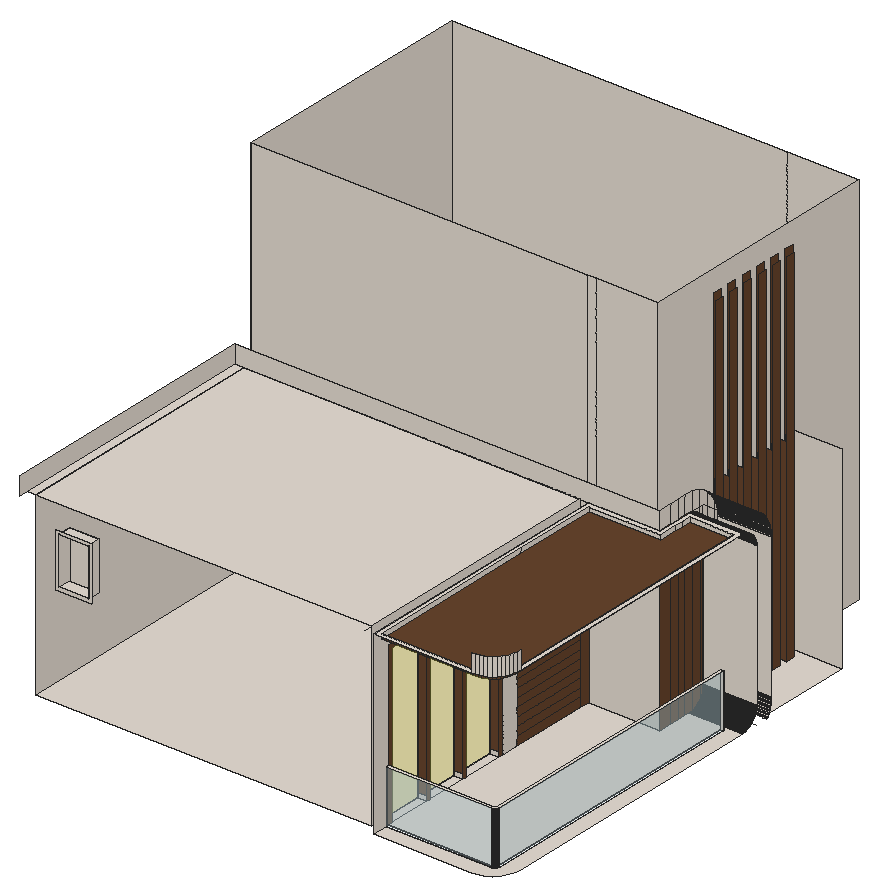
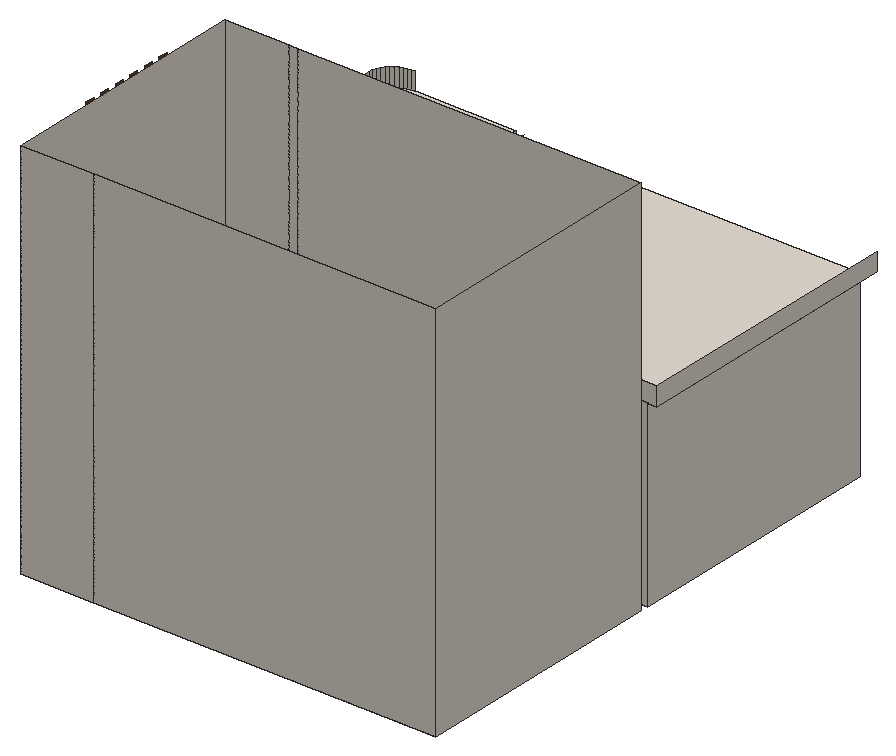
# SketchUp Ruby script. Lengths in inches.
U = 1.inch
M = Sketchup.active_model
def pt(a) = Geom::Point3d.new(a.map { |v| v * U })
def face(e, loops, mat)
  f = e.add_face(loops[0].map { |a| pt(a) })
  loops[1..].each { |l| e.add_face(l.map { |a| pt(a) }).erase! }
  f.material = f.back_material = mat if mat
  f
end
# faces: each face lists its corners as indices into pts; further lists are holes
def faces(e, pts, list, mat = nil) = list.each { |f| face(e, (f[0].is_a?(Array) ? f : [f]).map { |l| l.map { |i| pts[i] } }, mat) }
# xy, xz, yz: faces in a plane at the given z, y or x. An outline is a flat list of corners, or four numbers for a rectangle; further outlines are holes
def ring(l) = l.size == 4 ? [[l[0], l[1]], [l[2], l[1]], [l[2], l[3]], [l[0], l[3]]] : l.each_slice(2).to_a
def flat(e, list, mat, &to3) = list.each { |f| face(e, (f[0].is_a?(Array) ? f : [f]).map { |l| ring(l).map { |u, v| to3.(u, v) } }, mat) }
def xy(e, z, list, mat = nil) = flat(e, list, mat) { |x, y| [x, y, z] }
def xz(e, y, list, mat = nil) = flat(e, list, mat) { |x, z| [x, y, z] }
def yz(e, x, list, mat = nil) = flat(e, list, mat) { |y, z| [x, y, z] }
def lines(e, pts, list) = list.each { |a, b| e.add_line(pt(pts[a]), pt(pts[b])) }
# prism: a flat outline (further loops are holes) pulled along v
def prism(e, loops, v, mat = nil)
  f = face(e, loops, mat); d = Geom::Vector3d.new(v.map { |x| x * U })
  f.pushpull(f.normal.samedirection?(d) ? d.length : -d.length)
end
def box(e, o, s, mat = nil) = prism(e, [[o, [o[0] + s[0], o[1], o[2]], [o[0] + s[0], o[1] + s[1], o[2]], [o[0], o[1] + s[1], o[2]]]], [0, 0, s[2]], mat)
def at(x, y, z, deg = 0) = Geom::Transformation.translation(pt([x, y, z])) * Geom::Transformation.rotation(ORIGIN, Z_AXIS, deg.degrees)
def axes(o, x, y, z) = Geom::Transformation.new([*x, 0, *y, 0, *z, 0, *pt(o).to_a, 1])
def part(name) = M.definitions.add(name)
# library, detail: a bought-in or finely detailed component or shape, given as its bounding box
def library(name, o, s) = part(name).tap { |d| box(d.entities, o, s) }
def detail(e, o, s) = box(e.add_group.entities, o, s)
def put(e, d, t, mat = nil) = e.add_instance(d, t).tap { |i| i.material = mat if mat }
def group(e, t, mat = nil) = e.add_group.tap { |g| g.transformation = t; g.material = mat if mat }.entities
root = M.entities
M.materials.add("Glass_Basic_01").color = [255, 251, 32]
M.materials["Glass_Basic_01"].alpha = 0.25
M.materials.add("Glass_Safety_01").color = [204, 235, 244]
M.materials["Glass_Safety_01"].alpha = 0.25
M.materials.add("Marble_01_1K").color = [230, 221, 211]
M.materials.add("Wood_Veneer_15_1K").color = [103, 69, 45]
xy(root,132,[[273,36,339,36,341.36,36.13,343.68,36.57,345.92,37.3125,348.05,38.34,350.02,39.65,351.79,41.21,353.35,42.98,354.66,44.95,355.6875,47.08,356.43,49.32,356.87,51.64,357,54,357,240,321,240,321,216,273,216,273,48,344.08,48,344.21,48.02,344.33,48.0625,344.45,48.11,344.56,48.17,344.76,48.33,344.85,48.42,344.99,48.64,345.04,48.75,345.08,48.875,345.11,49,345.11,236.59,347.11,236.59,347.11,49,347.04,48.625,346.92,48.26,346.77,47.91,346.58,47.58,346.36,47.27,346.1,46.99,345.82,46.73,345.51,46.51,345.17,46.33,344.82,46.18,344.46,46.07,344.08,46,273,46],[42,42,267,216],[267,51,273,81],[267,83,273,111],[267,113,273,141],
  [42,222,315,390],[321,260.89,354,260.89,354,327,321,327,321,321,327,321,327,315,321,315,321,309,327,309,327,303,321,303,321,297,327,297,327,291,321,291,321,285,327,285,327,279,321,279,321,273,327,273,327,267,321,267],[321,267,327,273],[321,279,327,285],[321,291,327,297],
  [321,303,327,309],[321,315,327,321]],"Marble_01_1K")
xy(root,168,[[273,46,344.08,46,344.46,46.07,344.82,46.18,345.17,46.33,345.51,46.51,345.82,46.73,346.1,46.99,346.36,47.27,346.58,47.58,346.77,47.91,346.92,48.26,347.04,48.625,347.11,49,347.11,236.59,345.11,236.59,345.11,49,345.08,48.875,345.04,48.75,344.99,48.64,344.85,48.42,344.76,48.33,344.56,48.17,344.45,48.11,344.33,48.0625,344.21,48.02,344.08,48,273,48]],"Marble_01_1K")
xy(root,206,[[62,36,82,45]],"Marble_01_1K")
xy(root,237,[[267,51,273,81],[267,83,273,111],[267,113,273,141]],"Wood_Veneer_15_1K")
xy(root,238,[[62,36,82,45]],"Marble_01_1K")
xy(root,249,[[276,39,276,213,324,213,324,237,354,237,354,53.89,353.94,51.92,353.61,49.98,353.02,48.11,352.17,46.33,351.1,44.68,349.8,43.2,348.32,41.9,346.67,40.83,344.89,39.98,343.02,39.39,341.08,39.06,339.11,39]],"Wood_Veneer_15_1K")
xy(root,252,[[[273,36,273,216,321,216,321,240,357,240,357,54,356.92,51.62,356.53,49.28,355.81,47.01,354.79,44.86,353.49,42.87,351.92,41.08,350.13,39.51,348.14,38.21,345.99,37.19,343.72,36.47,341.38,36.08,339,36],[276,39,339.11,39,341.08,39.06,343.02,39.39,344.89,39.98,346.67,40.83,348.32,41.9,349.8,43.2,351.1,44.68,352.17,46.33,353.02,48.11,353.61,49.98,353.94,51.92,354,53.89,354,237,324,237,324,213,276,213]],[36,42,42,216],[42,42,267,216]],"Marble_01_1K")
xz(root,36,[[[60,204,84,240],[62,206,82,238]]],"Marble_01_1K")
xz(root,39,[[276,249,339.11,252]],"Wood_Veneer_15_1K")
xz(root,45,[[62,206,82,238]],"Marble_01_1K")
xz(root,46,[[273,132,344.08,168]],"Glass_Safety_01")
xz(root,48,[[273,132,344.08,168]],"Glass_Safety_01")
xz(root,51,[[267,132,273,135]],"Marble_01_1K")
xz(root,51,[[267,135,273,237]],"Wood_Veneer_15_1K")
xz(root,81,[[267,132,273,135]],"Marble_01_1K")
xz(root,81,[[267,135,273,237]],"Wood_Veneer_15_1K")
xz(root,83,[[267,132,273,135]],"Marble_01_1K")
xz(root,83,[[267,135,273,237]],"Wood_Veneer_15_1K")
xz(root,111,[[267,132,273,135]],"Marble_01_1K")
xz(root,111,[[267,135,273,237]],"Wood_Veneer_15_1K")
xz(root,113,[[267,132,273,135]],"Marble_01_1K")
xz(root,113,[[267,135,273,237]],"Wood_Veneer_15_1K")
xz(root,141,[[267,132,273,135]],"Marble_01_1K")
xz(root,141,[[267,135,273,237]],"Wood_Veneer_15_1K")
xz(root,213,[[276,249,324,252]],"Marble_01_1K")
xz(root,216,[[42,132,267,252],[273,132,321,252],[36,252,321,264]],"Marble_01_1K")
xz(root,222,[[42,132,267,384],[267,132,273,384],[273,132,315,384]],"Marble_01_1K")
xz(root,236.59,[[345.11,132,347.11,168]],"Marble_01_1K")
xz(root,237,[[324,249,354,252]],"Marble_01_1K")
xz(root,252,[[321,144,357,240]],"Marble_01_1K")
xz(root,261,[[321,251.14,327,264]],"Wood_Veneer_15_1K")
xz(root,264,[[321,143.24,357,144],[321,144,357,240]],"Marble_01_1K")
xz(root,267,[[321,132,327,264]],"Wood_Veneer_15_1K")
xz(root,273,[[321,132,327,264]],"Wood_Veneer_15_1K")
xz(root,279,[[321,132,327,264]],"Wood_Veneer_15_1K")
xz(root,285,[[321,132,327,264]],"Wood_Veneer_15_1K")
xz(root,291,[[321,132,327,264]],"Wood_Veneer_15_1K")
xz(root,297,[[321,132,327,264]],"Wood_Veneer_15_1K")
xz(root,303,[[321,132,327,264]],"Wood_Veneer_15_1K")
xz(root,309,[[321,132,327,264]],"Wood_Veneer_15_1K")
xz(root,315,[[321,132,327,264]],"Wood_Veneer_15_1K")
xz(root,321,[[321,132,327,264]],"Wood_Veneer_15_1K")
xz(root,327,[[321,132,354,264]],"Marble_01_1K")
xz(root,390,[[42,132,267,384],[267,132,315,384]],"Marble_01_1K")
yz(root,36,[[36,252,216,264]],"Marble_01_1K")
yz(root,42,[[42,132,216,252],[222,132,390,384]],"Marble_01_1K")
yz(root,62,[[36,206,45,238]],"Marble_01_1K")
yz(root,82,[[36,206,45,238]],"Marble_01_1K")
yz(root,267,[[51,132,81,237],[83,132,111,237],[113,132,141,237]],"Glass_Basic_01")
yz(root,267,[[42,132,42,252,216,252,216,132,141,132,141,237,113,237,113,132,111,132,111,237,83,237,83,132,81,132,81,237,51,237,51,132]],"Marble_01_1K")
yz(root,273,[[36,132,46,132,46,168,48,168,48,240,144,240,144,132,156,132,156,252,36,252]],"Marble_01_1K")
yz(root,273,[[48,132,51,132,51,237,141,237,141,132,144,132,144,240,48,240],[81,132,83,237],[111,132,113,237],[156,132,210,137.71],[210,132,216,132,216,252,156,252,156,246.26,210,246.26],
  [156,137.71,210,143.43],[156,143.43,210,149.14],[156,149.14,210,154.85],[156,154.85,210,160.56],[156,160.56,210,166.28],
  [156,166.28,210,171.99],[156,171.99,210,177.7],[156,177.7,210,183.42],[156,183.42,210,189.13],[156,189.13,210,194.84],
  [156,194.84,210,200.55],[156,200.55,210,206.27],[156,206.27,210,211.98],[156,211.98,210,217.69],[156,217.69,210,223.41],
  [156,223.41,210,229.12],[156,229.12,210,234.83],[156,234.83,210,240.55],[156,240.55,210,246.26]],"Wood_Veneer_15_1K")
yz(root,276,[[39,249,156,252],[156,249,213,252]],"Marble_01_1K")
yz(root,315,[[222,132,390,384]],"Marble_01_1K")
yz(root,321,[[252,132,255,132,255,258.4,254.54,258.77,253.95,259.22,253.34,259.65,252.71,260.07,252.08,260.46,251.43,260.84,250.77,261.2,250.11,261.54,249.43,261.85,249,262.04,249,252,252,252],[255,132,260.89,132,261,132.2,261,251.14,260.84,251.43,260.46,252.08,260.07,252.71,259.65,253.34,259.22,253.95,258.77,254.54,258.3,255.125,257.81,255.69,257.3,256.25,256.78,256.78,256.25,257.3,255.69,257.81,255.125,258.3,255,258.4],[260.89,132,261,132,261,132.2],[261,132.2,261.11,132.39,261.46,133.06,261.79,133.74,262.09,134.43,262.38,135.13,262.64,135.84,262.88,136.55,263.1,137.28,263.3,138.01,263.47,138.74,263.62,139.49,263.74,140.23,263.84,140.98,263.92,141.73,263.97,142.49,264,143.24,264,240,263.97,240.75,263.91,241.49,263.84,242.24,263.74,242.98,263.62,243.72,263.47,244.45,263.31,245.18,263.12,245.91,262.91,246.625,262.68,247.34,262.42,248.04,262.15,248.74,261.85,249.43,261.54,250.11,261.2,250.77,261,251.14],[216,252,225,264],
  [225,252,231,264],[231,252,237,264],[237,252,243,252,243,263.74,242.98,263.74,242.24,263.84,241.49,263.91,240.75,263.97,240,264,237,264],[243,252,249,252,249,262.04,248.74,262.15,248.04,262.42,247.34,262.68,246.625,262.91,245.91,263.12,245.18,263.31,244.45,263.47,243.72,263.62,243,263.74]],"Marble_01_1K")
yz(root,321,[[216,132,225,252],[225,132,231,252],[231,132,237,252],[237,132,240,132,240.37,132.02,241.11,132.1,241.48,132.16,241.85,132.23,242.21,132.3,242.57,132.39,242.93,132.49,243,132.51,243,251.26,242.83,251.32,242.49,251.4375,242.14,251.55,241.79,251.65,241.44,251.74,241.08,251.82,240.72,251.89,240.36,251.95,240,252,237,252],[261,132,267,132,267,375,261,375,261,251.14,261.2,250.77,261.54,250.11,261.85,249.43,262.15,248.74,262.42,248.04,262.68,247.34,262.91,246.625,263.12,245.91,263.31,245.18,263.47,244.45,263.62,243.72,263.74,242.98,263.84,242.24,263.91,241.49,263.97,240.75,264,240,264,143.24,263.97,142.49,263.92,141.73,263.84,140.98,263.74,140.23,263.62,139.49,263.47,138.74,263.3,138.01,263.1,137.28,262.88,136.55,262.64,135.84,262.38,135.13,262.09,134.43,261.79,133.74,261.46,133.06,261.11,132.39,261,132.2],
  [273,132,279,375],[285,132,291,375],[297,132,303,375],[309,132,315,375],[321,132,327,375],
  [243,132.51,243.29,132.6,243.64,132.72,243.99,132.85,244.33,132.99,244.67,133.14,245.01,133.3,245.34,133.47,245.66,133.65,245.98,133.84,246.3,134.04,246.61,134.25,246.91,134.47,247.2,134.69,247.78,135.17,248.05,135.42,248.32,135.68,248.58,135.95,248.83,136.22,249,136.42,249,246.97,248.78,247.24,248.54,247.51,248.29,247.78,248.04,248.04,247.78,248.29,247.51,248.54,247.24,248.78,246.95,249.02,246.67,249.24,246.375,249.46,246.08,249.67,245.77,249.875,245.47,250.07,244.83,250.43,244.51,250.6,243.85,250.92,243.52,251.06,243.18,251.2,243,251.26],[249,136.42,249.07,136.51,249.31,136.8,249.53,137.09,249.75,137.39,249.96,137.7,250.16,138.02,250.35,138.34,250.53,138.66,250.7,138.99,250.86,139.33,251.01,139.67,251.15,140.01,251.28,140.36,251.4,140.71,251.51,141.07,251.61,141.43,251.7,141.79,251.77,142.15,251.84,142.52,251.9,142.89,251.98,143.63,252,144,252,240,251.95,240.36,251.89,240.72,251.82,241.08,251.74,241.44,251.65,241.79,251.55,242.14,251.4375,242.49,251.32,242.83,251.2,243.18,251.06,243.52,250.92,243.85,250.6,244.51,250.43,244.83,250.07,245.47,249.875,245.77,249.67,246.08,249.46,246.375,249.24,246.67,249.02,246.95,249,246.97]],"Wood_Veneer_15_1K")
yz(root,324,[[213,249,225,252],[225,249,231,252],[231,249,237,252]],"Marble_01_1K")
yz(root,327,[[267,132,273,375],[279,132,285,375],[291,132,297,375],[303,132,309,375],[315,132,321,375],
  [261,251.14,261,375,255,375,255,258.4,255.125,258.3,255.69,257.81,256.25,257.3,256.78,256.78,257.3,256.25,257.81,255.69,258.3,255.125,258.77,254.54,259.22,253.95,259.65,253.34,260.07,252.71,260.46,252.08,260.84,251.43]],"Wood_Veneer_15_1K")
yz(root,345.11,[[49,132,236.59,168]],"Glass_Safety_01")
yz(root,347.11,[[49,132,236.59,168]],"Glass_Safety_01")
yz(root,354,[[53.89,249,237,252]],"Wood_Veneer_15_1K")
p = [[357,261.11,132.39],[357,260.89,132],[357,260.73,131.73],[354,260.73,131.73],[354,260.89,132],[321,260.89,132],
  [321,261,132.2],[321,261.11,132.39],[344.46,46.07,168],[344.08,46,168],[344.08,46,132],[344.46,46.07,132],
  [344.82,46.18,168],[344.82,46.18,132],[345.17,46.33,168],[345.17,46.33,132],[345.51,46.51,168],[345.51,46.51,132],
  [345.82,46.73,168],[345.82,46.73,132],[346.1,46.99,168],[346.1,46.99,132],[346.36,47.27,168],[346.36,47.27,132],
  [346.58,47.58,168],[346.58,47.58,132],[346.77,47.91,168],[346.77,47.91,132],[346.92,48.26,168],[346.92,48.26,132],
  [344.08,48,168],[344.21,48.02,168],[344.21,48.02,132],[344.08,48,132],[344.33,48.0625,168],[344.33,48.0625,132],
  [344.45,48.11,168],[344.45,48.11,132],[344.56,48.17,168],[344.56,48.17,132],[344.66,48.25,168],[344.66,48.25,132],
  [344.76,48.33,168],[344.76,48.33,132],[344.85,48.42,168],[344.85,48.42,132],[347.04,48.625,168],[347.04,48.625,132],
  [344.92,48.53,168],[344.92,48.53,132],[344.99,48.64,168],[344.99,48.64,132],[345.04,48.75,168],[345.04,48.75,132],
  [347.11,49,168],[347.11,49,132],[345.08,48.875,168],[345.08,48.875,132],[345.11,49,168],[345.11,49,132],
  [357,240,132],[357,240.37,132.02],[321,240.37,132.02],[321,240,132],[357,240.74,132.06],[321,240.74,132.06],
  [357,241.11,132.1],[321,241.11,132.1],[357,241.48,132.16],[321,241.48,132.16],[357,241.85,132.23],[321,241.85,132.23],
  [357,242.21,132.3],[321,242.21,132.3],[357,242.57,132.39],[321,242.57,132.39],[357,242.93,132.49],[321,242.93,132.49],
  [357,261.46,133.06],[321,261.46,133.06],[357,243.29,132.6],[321,243.29,132.6],[321,243,132.51],[357,243.64,132.72],
  [321,243.64,132.72],[357,243.99,132.85],[321,243.99,132.85],[357,244.33,132.99],[321,244.33,132.99],[357,244.67,133.14],
  [321,244.67,133.14],[357,245.01,133.3],[321,245.01,133.3],[357,261.79,133.74],[321,261.79,133.74],[357,245.34,133.47],
  [321,245.34,133.47],[357,245.66,133.65],[321,245.66,133.65],[357,245.98,133.84],[321,245.98,133.84],[357,262.09,134.43],
  [321,262.09,134.43],[357,246.3,134.04],[321,246.3,134.04],[357,246.61,134.25],[321,246.61,134.25],[357,246.91,134.47],
  [321,246.91,134.47],[357,262.38,135.13],[321,262.38,135.13],[357,247.2,134.69],[321,247.2,134.69],[357,247.49,134.93],
  [321,247.49,134.93],[357,247.78,135.17],[321,247.78,135.17],[357,262.64,135.84],[321,262.64,135.84],[357,248.05,135.42],
  [321,248.05,135.42],[357,248.32,135.68],[321,248.32,135.68],[357,248.58,135.95],[321,248.58,135.95],[357,262.88,136.55],
  [321,262.88,136.55],[357,248.83,136.22],[321,248.83,136.22],[357,249.07,136.51],[321,249.07,136.51],[321,249,136.42],
  [357,249.31,136.8],[321,249.31,136.8],[357,263.1,137.28],[321,263.1,137.28],[357,249.53,137.09],[321,249.53,137.09],
  [357,249.75,137.39],[321,249.75,137.39],[357,263.3,138.01],[321,263.3,138.01],[357,249.96,137.7],[321,249.96,137.7],
  [357,250.16,138.02],[321,250.16,138.02],[357,250.35,138.34],[321,250.35,138.34],[357,263.47,138.74],[321,263.47,138.74],
  [357,250.53,138.66],[321,250.53,138.66],[357,250.7,138.99],[321,250.7,138.99],[357,263.62,139.49],[321,263.62,139.49],
  [357,250.86,139.33],[321,250.86,139.33],[357,251.01,139.67],[321,251.01,139.67],[357,263.74,140.23],[321,263.74,140.23],
  [357,251.15,140.01],[321,251.15,140.01],[357,251.28,140.36],[321,251.28,140.36],[357,263.84,140.98],[321,263.84,140.98],
  [357,251.4,140.71],[321,251.4,140.71],[357,251.51,141.07],[321,251.51,141.07],[357,263.92,141.73],[321,263.92,141.73],
  [357,251.61,141.43],[321,251.61,141.43],[357,251.7,141.79],[321,251.7,141.79],[357,263.97,142.49],[321,263.97,142.49],
  [357,251.77,142.15],[321,251.77,142.15],[357,251.84,142.52],[321,251.84,142.52],[357,251.9,142.89],[321,251.9,142.89],
  [357,264,143.24],[321,264,143.24],[357,251.94,143.26],[321,251.94,143.26],[357,251.98,143.63],[321,251.98,143.63],
  [357,252,144],[321,252,144],[357,252,240],[357,251.95,240.36],[321,251.95,240.36],[321,252,240],
  [357,263.97,240.75],[357,264,240],[321,264,240],[321,263.97,240.75],[357,251.89,240.72],[321,251.89,240.72],
  [357,251.82,241.08],[321,251.82,241.08],[357,263.91,241.49],[321,263.91,241.49],[357,251.74,241.44],[321,251.74,241.44],
  [357,251.65,241.79],[321,251.65,241.79],[357,263.84,242.24],[321,263.84,242.24],[357,251.55,242.14],[321,251.55,242.14],
  [357,251.4375,242.49],[321,251.4375,242.49],[357,263.74,242.98],[321,263.74,242.98],[357,251.32,242.83],[321,251.32,242.83],
  [357,251.2,243.18],[321,251.2,243.18],[357,263.62,243.72],[321,263.62,243.72],[357,251.06,243.52],[321,251.06,243.52],
  [357,250.92,243.85],[321,250.92,243.85],[357,263.47,244.45],[321,263.47,244.45],[357,250.76,244.18],[321,250.76,244.18],
  [357,250.6,244.51],[321,250.6,244.51],[357,250.43,244.83],[321,250.43,244.83],[357,263.31,245.18],[321,263.31,245.18],
  [357,250.25,245.15],[321,250.25,245.15],[357,250.07,245.47],[321,250.07,245.47],[357,263.12,245.91],[321,263.12,245.91],
  [357,249.875,245.77],[321,249.875,245.77],[357,249.67,246.08],[321,249.67,246.08],[357,262.91,246.625],[321,262.91,246.625],
  [357,249.46,246.375],[321,249.46,246.375],[357,249.24,246.67],[321,249.24,246.67],[357,262.68,247.34],[321,262.68,247.34],
  [357,249.02,246.95],[321,249.02,246.95],[357,248.78,247.24],[321,248.78,247.24],[321,249,246.97],[357,248.54,247.51],
  [321,248.54,247.51],[357,262.42,248.04],[321,262.42,248.04],[357,248.29,247.78],[321,248.29,247.78],[357,248.04,248.04],
  [321,248.04,248.04],[357,247.78,248.29],[321,247.78,248.29],[357,262.15,248.74],[321,262.15,248.74],[357,247.51,248.54],
  [321,247.51,248.54],[357,247.24,248.78],[321,247.24,248.78],[357,261.85,249.43],[321,261.85,249.43],[357,246.95,249.02],
  [321,246.95,249.02],[341.08,39.06,252],[339.11,39,252],[339.11,39,249],[341.08,39.06,249],[343.02,39.39,252],
  [343.02,39.39,249],[344.89,39.98,252],[344.89,39.98,249],[346.67,40.83,252],[346.67,40.83,249],[348.32,41.9,252],
  [348.32,41.9,249],[349.8,43.2,252],[349.8,43.2,249],[351.1,44.68,252],[351.1,44.68,249],[352.17,46.33,252],
  [352.17,46.33,249],[353.02,48.11,252],[353.02,48.11,249],[353.61,49.98,252],[353.61,49.98,249],[353.94,51.92,252],
  [353.94,51.92,249],[354,53.89,252],[354,53.89,249],[357,246.67,249.24],[321,246.67,249.24],[357,246.375,249.46],
  [321,246.375,249.46],[357,261.54,250.11],[321,261.54,250.11],[357,246.08,249.67],[321,246.08,249.67],[357,245.77,249.875],
  [321,245.77,249.875],[357,245.47,250.07],[321,245.47,250.07],[357,245.15,250.25],[321,245.15,250.25],[357,261.2,250.77],
  [321,261.2,250.77],[357,244.83,250.43],[321,244.83,250.43],[357,244.51,250.6],[321,244.51,250.6],[357,244.18,250.76],
  [321,244.18,250.76],[357,243.85,250.92],[321,243.85,250.92],[357,260.84,251.43],[321,261,251.14],[327,261,251.14],
  [327,260.84,251.43],[357,243.52,251.06],[321,243.52,251.06],[357,243.18,251.2],[321,243.18,251.2],[321,260.84,251.43],
  [357,242.83,251.32],[321,242.83,251.32],[321,243,251.26],[357,242.49,251.4375],[321,242.49,251.4375],[357,242.14,251.55],
  [321,242.14,251.55],[321,260.46,252.08],[327,260.46,252.08],[357,260.46,252.08],[357,241.79,251.65],[321,241.79,251.65],
  [357,241.44,251.74],[321,241.44,251.74],[357,241.08,251.82],[321,241.08,251.82],[357,240.72,251.89],[321,240.72,251.89],
  [357,240.36,251.95],[357,240,252],[321,240,252],[321,240.36,251.95],[341.38,36.08,264],[339,36,264],
  [339,36,252],[341.38,36.08,252],[343.72,36.47,264],[343.72,36.47,252],[345.99,37.19,264],[345.99,37.19,252],
  [348.14,38.21,264],[348.14,38.21,252],[350.13,39.51,264],[350.13,39.51,252],[351.92,41.08,264],[351.92,41.08,252],
  [353.49,42.87,264],[353.49,42.87,252],[354.79,44.86,264],[354.79,44.86,252],[355.81,47.01,264],[355.81,47.01,252],
  [356.53,49.28,264],[356.53,49.28,252],[356.92,51.62,264],[356.92,51.62,252],[357,54,264],[357,54,252],
  [321,260.07,252.71],[327,260.07,252.71],[357,260.07,252.71],[321,259.65,253.34],[327,259.65,253.34],[357,259.65,253.34],
  [321,259.22,253.95],[327,259.22,253.95],[357,259.22,253.95],[321,258.77,254.54],[327,258.77,254.54],[357,258.77,254.54],
  [321,258.3,255.125],[327,258.3,255.125],[357,258.3,255.125],[321,257.81,255.69],[327,257.81,255.69],[357,257.81,255.69],
  [321,257.3,256.25],[327,257.3,256.25],[357,257.3,256.25],[321,256.78,256.78],[327,256.78,256.78],[357,256.78,256.78],
  [321,256.25,257.3],[327,256.25,257.3],[357,256.25,257.3],[321,255.69,257.81],[327,255.69,257.81],[357,255.69,257.81],
  [321,243,132],[357,252,132],[321,252,132],[357,252,252],[321,252,252],[321,249,132],
  [321,243,252],[321,249,252],[267,42,252],[267,36,252]]
faces(root,p,[[0,1,2,3,4,5,6,7],[60,61,62,63],[61,64,65,62],[64,66,67,65],[66,68,69,67],[68,70,71,69],[70,72,73,71],[72,74,75,73],
  [74,76,77,75],[78,0,7,79],[76,80,81,82,77],[80,83,84,81],[83,85,86,84],[85,87,88,86],[87,89,90,88],[89,91,92,90],
  [93,78,79,94],[91,95,96,92],[95,97,98,96],[97,99,100,98],[101,93,94,102],[99,103,104,100],[103,105,106,104],[105,107,108,106],
  [109,101,102,110],[107,111,112,108],[111,113,114,112],[113,115,116,114],[117,109,110,118],[115,119,120,116],[119,121,122,120],[121,123,124,122],
  [125,117,118,126],[123,127,128,124],[127,129,130,131,128],[129,132,133,130],[134,125,126,135],[132,136,137,133],[136,138,139,137],[140,134,135,141],
  [138,142,143,139],[142,144,145,143],[144,146,147,145],[148,140,141,149],[146,150,151,147],[150,152,153,151],[154,148,149,155],[152,156,157,153],
  [156,158,159,157],[160,154,155,161],[158,162,163,159],[162,164,165,163],[166,160,161,167],[164,168,169,165],[168,170,171,169],[172,166,167,173],
  [170,174,175,171],[174,176,177,175],[178,172,173,179],[176,180,181,177],[180,182,183,181],[182,184,185,183],[186,178,179,187],[184,188,189,185],
  [188,190,191,189],[190,192,193,191],[194,195,196,197],[198,199,200,201],[195,202,203,196],[202,204,205,203],[206,198,201,207],[204,208,209,205],
  [208,210,211,209],[212,206,207,213],[210,214,215,211],[214,216,217,215],[218,212,213,219],[216,220,221,217],[220,222,223,221],[224,218,219,225],
  [222,226,227,223],[226,228,229,227],[230,224,225,231],[228,232,233,229],[232,234,235,233],[234,236,237,235],[238,230,231,239],[236,240,241,237],
  [240,242,243,241],[244,238,239,245],[242,246,247,243],[246,248,249,247],[250,244,245,251],[248,252,253,249],[252,254,255,253],[256,250,251,257],
  [254,258,259,255],[258,260,261,262,259],[260,263,264,261],[265,256,257,266],[263,267,268,264],[267,269,270,268],[269,271,272,270],[273,265,266,274],
  [271,275,276,272],[275,277,278,276],[279,273,274,280],[277,281,282,278],[281,309,310,282],[309,311,312,310],[313,279,280,314],[311,315,316,312],
  [315,317,318,316],[317,319,320,318],[319,321,322,320],[323,313,314,324],[321,325,326,322],[325,327,328,326],[327,329,330,328],[329,331,332,330],
  [333,323,324,334,335,336],[331,337,338,332],[337,339,340,338],[334,341,336,335],[339,342,343,344,340],[342,345,346,343],[345,347,348,346],[341,349,350,336],
  [351,333,336,350],[347,352,353,348],[352,354,355,353],[354,356,357,355],[356,358,359,357],[360,361,362,363],[358,360,363,359],[364,365,366,367],
  [368,364,367,369],[370,368,369,371],[372,370,371,373],[374,372,373,375],[376,374,375,377],[378,376,377,379],[380,378,379,381],[382,380,381,383],
  [384,382,383,385],[386,384,385,387],[388,386,387,389],[349,390,391,350],[392,351,350,391],[390,393,394,391],[395,392,391,394],[393,396,397,394],
  [398,395,394,397],[396,399,400,397],[401,398,397,400],[399,402,403,400],[404,401,400,403],[402,405,406,403],[407,404,403,406],[405,408,409,406],
  [410,407,406,409],[408,411,412,409],[413,410,409,412],[411,414,415,412],[416,413,412,415],[414,417,418,415],[419,416,415,418]],"Marble_01_1K")
faces(root,p,[[8,9,10,11],[12,8,11,13],[14,12,13,15],[16,14,15,17],[18,16,17,19],[20,18,19,21],[22,20,21,23],[24,22,23,25],
  [26,24,25,27],[28,26,27,29],[30,31,32,33],[31,34,35,32],[34,36,37,35],[36,38,39,37],[38,40,41,39],[40,42,43,41],
  [42,44,45,43],[46,28,29,47],[44,48,49,45],[48,50,51,49],[50,52,53,51],[54,46,47,55],[52,56,57,53],[56,58,59,57]],"Glass_Safety_01")
faces(root,p,[[283,284,285,286],[287,283,286,288],[289,287,288,290],[291,289,290,292],[293,291,292,294],[295,293,294,296],[297,295,296,298],[299,297,298,300],
  [301,299,300,302],[303,301,302,304],[305,303,304,306],[307,305,306,308]],"Wood_Veneer_15_1K")
lines(root,p,[[63,420],[421,422],[423,424],[420,425],[344,426],[420,82],[425,131],[425,422],[262,427],[428,429]])
